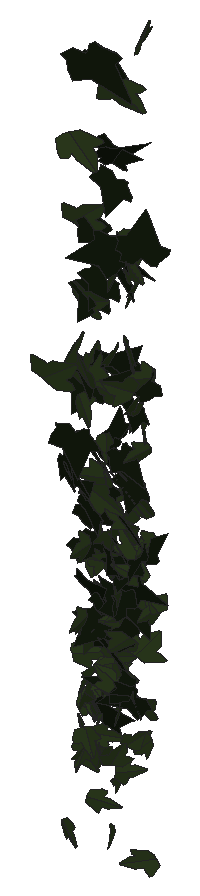
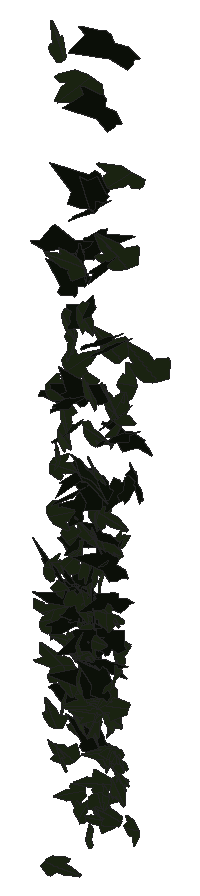
# SketchUp Ruby script. Lengths in inches.
U = 1.inch
M = Sketchup.active_model
def pt(a) = Geom::Point3d.new(a.map { |v| v * U })
def face(e, loops, mat)
  f = e.add_face(loops[0].map { |a| pt(a) })
  loops[1..].each { |l| e.add_face(l.map { |a| pt(a) }).erase! }
  f.material = f.back_material = mat if mat
  f
end
# faces: each face lists its corners as indices into pts; further lists are holes
def faces(e, pts, list, mat = nil) = list.each { |f| face(e, (f[0].is_a?(Array) ? f : [f]).map { |l| l.map { |i| pts[i] } }, mat) }
# xy, xz, yz: faces in a plane at the given z, y or x. An outline is a flat list of corners, or four numbers for a rectangle; further outlines are holes
def ring(l) = l.size == 4 ? [[l[0], l[1]], [l[2], l[1]], [l[2], l[3]], [l[0], l[3]]] : l.each_slice(2).to_a
def flat(e, list, mat, &to3) = list.each { |f| face(e, (f[0].is_a?(Array) ? f : [f]).map { |l| ring(l).map { |u, v| to3.(u, v) } }, mat) }
def xy(e, z, list, mat = nil) = flat(e, list, mat) { |x, y| [x, y, z] }
def xz(e, y, list, mat = nil) = flat(e, list, mat) { |x, z| [x, y, z] }
def yz(e, x, list, mat = nil) = flat(e, list, mat) { |y, z| [x, y, z] }
def lines(e, pts, list) = list.each { |a, b| e.add_line(pt(pts[a]), pt(pts[b])) }
# prism: a flat outline (further loops are holes) pulled along v
def prism(e, loops, v, mat = nil)
  f = face(e, loops, mat); d = Geom::Vector3d.new(v.map { |x| x * U })
  f.pushpull(f.normal.samedirection?(d) ? d.length : -d.length)
end
def box(e, o, s, mat = nil) = prism(e, [[o, [o[0] + s[0], o[1], o[2]], [o[0] + s[0], o[1] + s[1], o[2]], [o[0], o[1] + s[1], o[2]]]], [0, 0, s[2]], mat)
def at(x, y, z, deg = 0) = Geom::Transformation.translation(pt([x, y, z])) * Geom::Transformation.rotation(ORIGIN, Z_AXIS, deg.degrees)
def axes(o, x, y, z) = Geom::Transformation.new([*x, 0, *y, 0, *z, 0, *pt(o).to_a, 1])
def part(name) = M.definitions.add(name)
# library, detail: a bought-in or finely detailed component or shape, given as its bounding box
def library(name, o, s) = part(name).tap { |d| box(d.entities, o, s) }
def detail(e, o, s) = box(e.add_group.entities, o, s)
def put(e, d, t, mat = nil) = e.add_instance(d, t).tap { |i| i.material = mat if mat }
def group(e, t, mat = nil) = e.add_group.tap { |g| g.transformation = t; g.material = mat if mat }.entities
root = M.entities
M.materials.add("1026 AP 7946 SUNNY SIDE UP").color = [254, 231, 186]
M.materials.add("efeu1").color = [18, 25, 13]
M.materials.add("efeu2").color = [43, 57, 29]
c1 = part("ivyleaf_10")
p = [[0,0.5,-0.03],[-0.0625,2.02,-0.43],[-0.19,2.01,-0.46],[-0.54,1.05,-0.29],[-0.52,0.625,-0.18],[-0.83,0.76,-0.28],
  [-1.16,0.64,-0.33],[-1.15,0.33,-0.24],[-0.77,-0.39,0.02],[-0.3,-0.51,0.16],[0.04,-0.48,0.23],[-0.02,2.01,-0.4375],
  [-0.06,2.01,-0.43],[0.04,-0.49,0.23],[0.67,-0.49,0.14],[1.38,0.36,-0.2],[1.375,0.51,-0.24],[0.81,0.65,-0.19],
  [0.62,0.59,-0.15],[0.6,1.09,-0.28],[0.5,1.23,-0.31]]
faces(c1.entities,p,[[0,1,2,3,4,5,6,7,8,9,10],[11,12,0,13,14,15,16,17,18,19,20]],"efeu2")
c2 = part("ivyleaf_9")
p = [[1.54,2.16,1.25],[1.36,2.04,1.19],[-0.21,0.99,0.68],[-0.71,1.11,0.82],[-0.85,0.86,0.67],[-0.8,0.17,0.21],
  [-0.9,-0.01,0.1],[-0.67,-0.16,-0.02],[-0.08,-0.08,-0.05],[-0.03,-0.6,-0.4],[0.65,-0.88,-0.66],[0.83,-0.6,-0.49],
  [1.29,-0.42,-0.43],[1.8125,-0.07,-0.26],[1.21,0.44,0.15]]
faces(c2.entities,p,[[0,1,2,3,4,5,6,7,8,9,10,11,12,13,14]],"efeu1")
put(root,c1,axes([104.67,210.25,259.6],[-0.39071,-0.04225,0.21205],[0.30866,0.06806,0.25862],[-0.11888,0.31556,-0.02542]),"1026 AP 7946 SUNNY SIDE UP")
put(root,c1,axes([104.85,210.58,248.98],[-0.13045,0.07841,-0.19526],[0.16908,-0.15804,-0.1165],[-0.27541,-0.13416,0.02097]),"1026 AP 7946 SUNNY SIDE UP")
put(root,c2,axes([105.08,210.6,258.22],[-0.31451,-0.09252,-0.20284],[0.30315,0.047,-0.22484],[0.15687,-0.27633,0.02783]),"1026 AP 7946 SUNNY SIDE UP")
put(root,c1,axes([105.19,210.78,255.5625],[-0.0292,0.01458,0.27031],[0.11932,-0.25145,0.01847],[0.39547,0.07694,0.01439]),"1026 AP 7946 SUNNY SIDE UP")
put(root,c2,axes([105.41,210.61,267.22],[-0.07439,-0.12984,-0.33099],[0.41359,0.19657,-0.12086],[0.35311,-0.25759,0.07184]),"1026 AP 7946 SUNNY SIDE UP")
put(root,c1,axes([106.08,210.62,250.9],[-0.19009,-0.18862,0.0504],[0.02785,0.04797,0.23082],[-0.30557,0.12171,-0.01032]),"1026 AP 7946 SUNNY SIDE UP")
put(root,c1,axes([106.22,210.9,259.51],[-0.09492,-0.10563,-0.25333],[-0.24533,-0.19017,0.1228],[-0.34084,0.16629,-0.01784]),"1026 AP 7946 SUNNY SIDE UP")
put(root,c2,axes([104.53,210.9,257.35],[-0.01055,-0.07019,-0.26013],[0.39949,-0.06221,0.01051],[-0.09865,-0.2444,0.07039]),"1026 AP 7946 SUNNY SIDE UP")
put(root,c1,axes([105.5,210.8,256.85],[0.07563,0.0111,0.27061],[0.41267,-0.01686,-0.04888],[0.02296,0.26645,-0.0128]),"1026 AP 7946 SUNNY SIDE UP")
put(root,c2,axes([105.71,211.02,262.58],[-0.01995,-0.17839,-0.27056],[0.05025,-0.26121,0.18036],[-0.49535,-0.01931,0.02919]),"1026 AP 7946 SUNNY SIDE UP")
put(root,c2,axes([104.72,210.85,257.2],[0.2917,-0.16938,-0.08061],[-0.10055,0.0445,-0.25833],[0.27493,0.19598,-0.00895]),"1026 AP 7946 SUNNY SIDE UP")
put(root,c1,axes([105.6,211.15,248.78],[0.01372,-0.00257,0.2245],[0.18259,-0.18452,-0.00811],[0.29002,0.1163,-0.00551]),"1026 AP 7946 SUNNY SIDE UP")
put(root,c1,axes([104.72,211.27,253.47],[0.00942,-0.01726,0.24563],[0.11612,-0.22681,-0.02015],[0.35767,0.07409,0.00007]),"1026 AP 7946 SUNNY SIDE UP")
put(root,c1,axes([104.9,211.15,250.91],[0.28899,-0.02084,0.13185],[0.19382,-0.0415,-0.18938],[0.06389,0.22015,-0.02187]),"1026 AP 7946 SUNNY SIDE UP")
put(root,c1,axes([104.86,211.15,250.57],[0.28019,-0.1356,0.01598],[0.00399,-0.02348,-0.23015],[0.21472,0.17739,-0.01658]),"1026 AP 7946 SUNNY SIDE UP")
put(root,c1,axes([105.77,211.08,266.39],[-0.37776,-0.1049,-0.18914],[0.27999,0.04784,-0.26879],[0.17781,-0.29819,0.02141]),"1026 AP 7946 SUNNY SIDE UP")
put(root,c1,axes([104.83,211.125,258.67],[-0.03331,0.2618,0.0245],[-0.00537,0.0221,-0.27045],[-0.41311,-0.02139,0.00154]),"1026 AP 7946 SUNNY SIDE UP")
put(root,c1,axes([106.01,211.14,260.35],[-0.23991,0.22338,0.0069],[-0.02477,-0.00419,-0.27825],[-0.35047,-0.15261,0.01494]),"1026 AP 7946 SUNNY SIDE UP")
put(root,c2,axes([106.13,211.23,252.16],[0.02174,-0.00557,-0.25392],[-0.30638,-0.15144,-0.00862],[-0.23742,0.19492,-0.01212]),"1026 AP 7946 SUNNY SIDE UP")
put(root,c1,axes([104.59,211.03,259.67],[0.10621,-0.15859,0.25953],[-0.13424,0.23812,0.17877],[-0.44967,-0.10854,0.00793]),"1026 AP 7946 SUNNY SIDE UP")
put(root,c1,axes([104.57,211.18,264.68],[0.33939,0.14432,0.17421],[0.24991,0.06302,-0.2653],[-0.24303,0.26634,-0.02953]),"1026 AP 7946 SUNNY SIDE UP")
put(root,c1,axes([104.77,211.3,250.38],[0.01574,-0.23389,0.04801],[0.00412,-0.04787,-0.24145],[0.37538,0.01033,0.00064]),"1026 AP 7946 SUNNY SIDE UP")
put(root,c1,axes([104.92,211.125,251.86],[0.00604,-0.15577,-0.18379],[0.04217,0.17668,-0.15808],[0.36895,-0.01765,0.02108]),"1026 AP 7946 SUNNY SIDE UP")
put(root,c1,axes([105.82,211.31,253.35],[-0.24966,-0.07644,0.13494],[-0.16673,-0.08049,-0.18069],[0.17132,-0.18974,0.0208]),"1026 AP 7946 SUNNY SIDE UP")
put(root,c1,axes([105.56,211.31,252.22],[0.14756,0.18616,0.1326],[-0.10792,-0.10817,0.21385],[0.33812,-0.11576,0.01039]),"1026 AP 7946 SUNNY SIDE UP")
put(root,c1,axes([105.05,211.24,249.4],[-0.03261,-0.03409,-0.20746],[0.31874,0.01972,-0.02485],[0.03675,-0.20129,0.03147]),"1026 AP 7946 SUNNY SIDE UP")
put(root,c2,axes([105.83,211.27,252.21],[-0.24014,0.0961,0.17319],[-0.24571,0.0641,-0.18422],[-0.17854,-0.21747,0.0206]),"1026 AP 7946 SUNNY SIDE UP")
put(root,c1,axes([106.15,211.21,252.0625],[-0.1781,0.18411,0.12725],[-0.12095,0.09621,-0.22171],[-0.32598,-0.13629,0.01274]),"1026 AP 7946 SUNNY SIDE UP")
put(root,c1,axes([104.76,211.32,259.1],[-0.39005,0.11307,-0.08509],[-0.10168,0.05798,0.28002],[0.19596,0.25515,-0.02406]),"1026 AP 7946 SUNNY SIDE UP")
put(root,c2,axes([105.47,211.51,262.44],[0.04387,-0.07054,-0.26418],[0.3938,-0.07866,0.04998],[-0.13892,-0.24524,0.05826]),"1026 AP 7946 SUNNY SIDE UP")
put(root,c1,axes([105.58,211.51,251.76],[0.15613,-0.15263,0.183],[0.12893,-0.15908,-0.18804],[0.34606,0.12813,-0.01251]),"1026 AP 7946 SUNNY SIDE UP")
put(root,c1,axes([105.76,211.5,262.06],[-0.10086,0.00186,-0.26934],[0.24674,-0.21506,-0.04249],[-0.32885,-0.16193,0.05073]),"1026 AP 7946 SUNNY SIDE UP")
put(root,c1,axes([105.34,211.46,252.43],[0.25706,-0.08457,0.11464],[0.14138,-0.06843,-0.18924],[0.16904,0.18583,-0.01606]),"1026 AP 7946 SUNNY SIDE UP")
put(root,c1,axes([104.74,211.55,252.11],[0.06146,-0.1705,0.16311],[0.04199,-0.15719,-0.18099],[0.36449,0.04686,-0.00665]),"1026 AP 7946 SUNNY SIDE UP")
put(root,c1,axes([104.57,211.36,262.75],[-0.32078,-0.12877,0.17326],[0.19886,0.11452,0.24796],[-0.26831,0.23882,-0.02336]),"1026 AP 7946 SUNNY SIDE UP")
put(root,c2,axes([105.34,211.54,252.75],[0.21758,-0.21418,0.00234],[0.01628,0.01083,0.26232],[-0.33643,-0.13799,0.0142]),"1026 AP 7946 SUNNY SIDE UP")
put(root,c1,axes([104.51,211.47,250.96],[-0.11372,0.15878,-0.10474],[0.05418,-0.09691,-0.18014],[-0.29225,-0.07975,0.00736]),"1026 AP 7946 SUNNY SIDE UP")
put(root,c1,axes([105.09,211.53,257.7],[0.23289,-0.0714,0.14625],[0.17784,-0.08975,-0.1681],[0.17634,0.1848,-0.02363]),"1026 AP 7946 SUNNY SIDE UP")
put(root,c2,axes([105.11,211.51,251.24],[0.0382,-0.00478,0.25809],[0.2486,-0.19502,-0.02077],[0.30573,0.15917,-0.01536]),"1026 AP 7946 SUNNY SIDE UP")
put(root,c2,axes([105.8,211.61,256.9],[-0.09049,-0.23355,0.08295],[-0.01312,-0.08215,-0.24803],[0.38892,-0.05712,0.01093]),"1026 AP 7946 SUNNY SIDE UP")
put(root,c2,axes([105.29,211.63,263.78],[-0.11668,-0.25223,0.08957],[-0.01872,-0.08851,-0.27105],[0.41983,-0.07405,0.01281]),"1026 AP 7946 SUNNY SIDE UP")
put(root,c2,axes([106.21,211.33,262.48],[-0.40718,-0.04558,0.17485],[0.25155,0.06504,0.26943],[-0.11531,0.30286,-0.02965]),"1026 AP 7946 SUNNY SIDE UP")
put(root,c1,axes([104.8125,211.42,259.26],[0.39193,-0.17902,0.03078],[-0.01704,0.03771,0.31539],[-0.28515,-0.24832,0.02346]),"1026 AP 7946 SUNNY SIDE UP")
put(root,c2,axes([104.8125,211.48,262.68],[0.07366,-0.2428,-0.1194],[-0.03524,0.11231,-0.25409],[0.42065,0.05193,-0.00038]),"1026 AP 7946 SUNNY SIDE UP")
put(root,c1,axes([105.68,211.58,255.97],[-0.16017,-0.08066,-0.19101],[-0.25573,-0.08981,0.1321],[-0.18779,0.1911,-0.01698]),"1026 AP 7946 SUNNY SIDE UP")
put(root,c1,axes([105.06,211.58,251.47],[0.1803,-0.17179,0.08103],[0.05117,-0.07383,-0.21279],[0.2933,0.11848,-0.01269]),"1026 AP 7946 SUNNY SIDE UP")
put(root,c2,axes([104.5,211.65,259.19],[0.01047,-0.24314,0.07181],[0.01163,-0.07089,-0.25094],[0.39815,0.00846,0.00544]),"1026 AP 7946 SUNNY SIDE UP")
put(root,c1,axes([105.41,211.64,254.18],[-0.10344,0.08288,0.2105],[0.15793,-0.17801,0.1069],[0.30788,0.11916,0.01588]),"1026 AP 7946 SUNNY SIDE UP")
put(root,c2,axes([105.82,211.46,253.35],[-0.26131,0.15261,0.1024],[-0.13415,0.05233,-0.23142],[-0.25216,-0.18597,0.017]),"1026 AP 7946 SUNNY SIDE UP")
put(root,c2,axes([105.7,211.43,254.03],[-0.34158,-0.01045,-0.13283],[-0.20328,0.02189,0.2228],[0.00349,0.25164,-0.02341]),"1026 AP 7946 SUNNY SIDE UP")
put(root,c2,axes([104.61,211.6875,255.93],[0.03816,-0.20861,0.13079],[0.03687,-0.1262,-0.21696],[0.38319,0.03291,0.00785]),"1026 AP 7946 SUNNY SIDE UP")
put(root,c1,axes([104.49,211.66,253.22],[-0.01141,0.0825,-0.19897],[0.00016,-0.19372,-0.08618],[-0.33092,-0.00294,0.00682]),"1026 AP 7946 SUNNY SIDE UP")
put(root,c2,axes([104.97,211.67,253.32],[-0.34817,-0.11962,0.03396],[-0.02695,-0.03869,-0.25815],[0.19353,-0.2206,0.02515]),"1026 AP 7946 SUNNY SIDE UP")
put(root,c2,axes([104.53,211.71,258.74],[-0.18887,-0.21888,0.08833],[-0.03569,-0.08643,-0.25685],[0.36863,-0.12051,0.02038]),"1026 AP 7946 SUNNY SIDE UP")
put(root,c2,axes([105.47,211.64,256],[0.17146,-0.20273,0.09806],[0.06338,-0.08767,-0.23759],[0.34719,0.11612,-0.00506]),"1026 AP 7946 SUNNY SIDE UP")
put(root,c2,axes([105.4,211.64,256.71],[0.21199,-0.17618,0.12948],[0.09275,-0.11377,-0.22834],[0.32836,0.14588,-0.01909]),"1026 AP 7946 SUNNY SIDE UP")
put(root,c2,axes([105.21,211.72,254.8],[0.17525,-0.13069,-0.18207],[0.19656,-0.1243,0.17591],[-0.28315,-0.16717,0.00943]),"1026 AP 7946 SUNNY SIDE UP")
put(root,c1,axes([105.65,211.58,255.7],[-0.24117,0.05716,0.14748],[0.2179,-0.03627,0.16804],[0.10507,0.20642,-0.00997]),"1026 AP 7946 SUNNY SIDE UP")
put(root,c1,axes([105.02,211.57,256.78],[-0.1124,-0.00188,0.24224],[-0.35248,-0.0737,-0.07124],[0.1117,-0.23446,0.01894]),"1026 AP 7946 SUNNY SIDE UP")
put(root,c1,axes([105.98,211.6,267.26],[0.11827,-0.29639,-0.05099],[0.02936,-0.04458,0.31468],[-0.47116,-0.07718,0.00681]),"1026 AP 7946 SUNNY SIDE UP")
put(root,c2,axes([105.5,211.68,262.01],[0.11049,-0.13601,0.23014],[0.22824,-0.17309,-0.15608],[0.34335,0.15883,0.02969]),"1026 AP 7946 SUNNY SIDE UP")
put(root,c1,axes([104.51,211.59,260.71],[-0.25667,0.01621,0.23957],[0.36576,-0.00551,0.16863],[0.02174,0.28399,-0.00873]),"1026 AP 7946 SUNNY SIDE UP")
put(root,c1,axes([106.16,211.63,248.18],[0.15677,0.0237,-0.20343],[-0.29206,-0.06831,-0.10538],[-0.11241,0.21053,-0.00991]),"1026 AP 7946 SUNNY SIDE UP")
put(root,c1,axes([106.06,211.74,259.39],[0.00268,0.0483,0.256],[-0.01027,-0.24813,0.04834],[0.39749,-0.00674,-0.00047]),"1026 AP 7946 SUNNY SIDE UP")
put(root,c2,axes([104.85,211.69,257.21],[0.1503,-0.15026,0.19586],[0.16935,-0.15777,-0.18433],[0.34251,0.14394,0.00519]),"1026 AP 7946 SUNNY SIDE UP")
put(root,c1,axes([105.91,211.55,258.91],[0.03799,-0.26106,-0.07214],[-0.01595,0.06789,-0.26967],[0.42411,0.02594,-0.00368]),"1026 AP 7946 SUNNY SIDE UP")
put(root,c2,axes([106.09,211.72,259.35],[-0.06432,-0.12249,-0.22488],[-0.15798,-0.19379,0.1307],[-0.35945,0.10709,-0.0172]),"1026 AP 7946 SUNNY SIDE UP")
put(root,c1,axes([105.87,211.66,254.68],[0.10562,0.09858,0.19017],[-0.19959,-0.13421,0.121],[0.26064,-0.14272,0.0156]),"1026 AP 7946 SUNNY SIDE UP")
put(root,c2,axes([104.47,211.67,257.42],[0.25226,-0.2001,0.04438],[0.0214,-0.04562,-0.26386],[0.32152,0.16003,-0.01725]),"1026 AP 7946 SUNNY SIDE UP")
put(root,c1,axes([105.25,211.63,259.76],[0.0692,-0.26731,0.00468],[-0.00569,-0.00673,-0.27909],[0.42039,0.04391,-0.00455]),"1026 AP 7946 SUNNY SIDE UP")
put(root,c2,axes([105.51,211.58,257.51],[0.08607,-0.20152,-0.15844],[-0.04183,0.15073,-0.21394],[0.39532,0.05982,0.01186]),"1026 AP 7946 SUNNY SIDE UP")
put(root,c2,axes([104.63,211.82,260.86],[-0.17164,-0.21798,0.12258],[-0.04753,-0.1187,-0.25068],[0.38853,-0.11082,0.02349]),"1026 AP 7946 SUNNY SIDE UP")
put(root,c1,axes([105.94,211.77,257.65],[-0.02414,-0.09557,0.19933],[-0.04813,-0.1916,-0.10084],[0.33668,-0.03424,-0.00012]),"1026 AP 7946 SUNNY SIDE UP")
put(root,c1,axes([105.53,211.68,262.46],[-0.08159,-0.01667,-0.27051],[0.38147,-0.10639,-0.04307],[-0.15976,-0.24551,0.03532]),"1026 AP 7946 SUNNY SIDE UP")
put(root,c2,axes([105.28,211.57,259.36],[-0.18533,-0.01149,0.24255],[0.36954,-0.02706,0.11965],[0.03004,0.26197,0.02455]),"1026 AP 7946 SUNNY SIDE UP")
put(root,c1,axes([106.13,211.6,256.35],[-0.20303,0.05043,-0.17723],[-0.24993,0.0666,0.14317],[0.13129,0.20477,-0.00152]),"1026 AP 7946 SUNNY SIDE UP")
put(root,c2,axes([105.54,211.73,254.95],[-0.32893,-0.07376,-0.10427],[0.16135,0.0106,-0.22733],[0.11197,-0.23197,0.02127]),"1026 AP 7946 SUNNY SIDE UP")
put(root,c2,axes([104.52,211.76,253.89],[-0.07811,-0.04816,0.24698],[0.20339,-0.21309,-0.01772],[0.3268,0.12111,0.07005]),"1026 AP 7946 SUNNY SIDE UP")
put(root,c1,axes([105.77,211.58,250.79],[-0.13261,-0.13051,0.13696],[0.09307,0.12046,0.16032],[-0.27865,0.10235,-0.01163]),"1026 AP 7946 SUNNY SIDE UP")
put(root,c2,axes([105.24,211.82,255.13],[0.00292,-0.1314,0.22313],[0.0885,-0.21173,-0.1336],[0.38941,0.0491,0.02869]),"1026 AP 7946 SUNNY SIDE UP")
put(root,c1,axes([106.12,211.64,250.93],[0.21967,-0.15689,-0.09427],[-0.11693,0.05469,-0.21534],[0.25978,0.15728,-0.01721]),"1026 AP 7946 SUNNY SIDE UP")
put(root,c1,axes([105.35,211.78,253.4375],[-0.01498,0.04787,0.2089],[-0.07479,-0.19786,0.04472],[0.31854,-0.0442,0.02032]),"1026 AP 7946 SUNNY SIDE UP")
put(root,c2,axes([105.68,211.68,254.07],[-0.02695,-0.21843,-0.13728],[0.04767,0.12964,-0.22426],[0.39848,-0.03028,0.01754]),"1026 AP 7946 SUNNY SIDE UP")
put(root,c1,axes([106.16,211.84,253.94],[-0.05313,-0.02706,0.23788],[0.04987,-0.23184,-0.02455],[0.36239,0.02794,0.03826]),"1026 AP 7946 SUNNY SIDE UP")
put(root,c1,axes([105.3,211.82,249.7],[-0.03522,-0.06502,-0.2015],[-0.04332,-0.19366,0.06857],[-0.32064,0.03331,0.01287]),"1026 AP 7946 SUNNY SIDE UP")
put(root,c2,axes([105.59,211.67,254.42],[0.16562,-0.01763,-0.22767],[0.31958,0.10515,0.09181],[0.13886,-0.22098,0.06026]),"1026 AP 7946 SUNNY SIDE UP")
put(root,c1,axes([105.46,211.8125,253.62],[-0.0232,-0.04882,0.20844],[-0.07414,-0.19707,-0.05361],[0.31921,-0.04932,0.0027]),"1026 AP 7946 SUNNY SIDE UP")
put(root,c2,axes([104.82,211.7,256.42],[-0.15752,-0.07194,-0.22236],[0.30103,0.09995,-0.12551],[0.19217,-0.21554,0.01435]),"1026 AP 7946 SUNNY SIDE UP")
put(root,c2,axes([105.63,211.86,258.53],[-0.04582,-0.19985,0.14158],[0.02195,-0.1407,-0.20685],[0.38175,-0.0159,0.02889]),"1026 AP 7946 SUNNY SIDE UP")
put(root,c1,axes([104.87,211.81,256.74],[-0.00763,-0.009,0.21925],[0.22381,-0.15859,-0.00449],[0.24931,0.14209,0.01074]),"1026 AP 7946 SUNNY SIDE UP")
put(root,c1,axes([104.66,211.64,251.35],[-0.26892,0.14404,0.02674],[-0.04963,0.0014,-0.22949],[-0.22449,-0.17286,0.0187]),"1026 AP 7946 SUNNY SIDE UP")
put(root,c1,axes([105.16,211.66,255.48],[-0.1029,-0.23676,-0.05125],[0.02499,0.04582,-0.25277],[0.37916,-0.06728,0.00275]),"1026 AP 7946 SUNNY SIDE UP")
put(root,c2,axes([105.36,211.65,257.74],[-0.22547,0.2023,-0.00715],[-0.01055,-0.01465,-0.25514],[-0.31818,-0.14287,0.01352]),"1026 AP 7946 SUNNY SIDE UP")
put(root,c1,axes([105.77,211.7,255.25],[0.19137,0.22637,0.07581],[-0.07945,-0.05473,0.26381],[0.36511,-0.13056,0.01767]),"1026 AP 7946 SUNNY SIDE UP")
put(root,c1,axes([106.02,211.72,251.6],[-0.28979,0.04874,0.10891],[0.16925,-0.00272,0.19509],[0.06869,0.21231,-0.0212]),"1026 AP 7946 SUNNY SIDE UP")
put(root,c1,axes([105.04,211.66,252.3],[-0.1436,-0.05156,-0.23233],[0.35461,0.0328,-0.10175],[0.07904,-0.24082,0.03438]),"1026 AP 7946 SUNNY SIDE UP")
put(root,c1,axes([105.51,211.5625,250.06],[-0.00453,-0.02696,-0.22851],[0.22295,0.17103,-0.02233],[0.27123,-0.14104,0.01453]),"1026 AP 7946 SUNNY SIDE UP")
put(root,c2,axes([105.73,211.8,255.29],[-0.27608,0.00545,-0.17906],[0.26883,-0.03998,-0.17941],[-0.05024,-0.24382,0.02395]),"1026 AP 7946 SUNNY SIDE UP")
put(root,c1,axes([104.4,211.59,252.43],[0.07217,-0.00443,-0.23803],[0.30938,0.12427,0.03854],[0.19053,-0.2001,0.02758]),"1026 AP 7946 SUNNY SIDE UP")
put(root,c1,axes([104.38,211.76,251.22],[0.11777,0.0083,0.21208],[0.32055,-0.03437,-0.0752],[0.04641,0.21631,-0.01879]),"1026 AP 7946 SUNNY SIDE UP")
put(root,c1,axes([105.05,211.74,256.24],[0.21336,-0.08832,-0.14337],[0.20079,-0.05662,0.16555],[-0.16281,-0.18556,0.01629]),"1026 AP 7946 SUNNY SIDE UP")
put(root,c1,axes([104.92,211.79,256.33],[0.17234,-0.18381,0.05971],[0.0268,-0.05837,-0.22029],[0.30236,0.10994,-0.01451]),"1026 AP 7946 SUNNY SIDE UP")
put(root,c1,axes([104.85,211.74,250.22],[-0.1615,-0.19463,0.02244],[-0.00208,-0.02515,-0.2266],[0.30813,-0.10218,0.01023]),"1026 AP 7946 SUNNY SIDE UP")
put(root,c2,axes([105.04,211.62,264.28],[0.25363,0.22666,-0.07874],[0.04771,0.07361,0.28647],[0.37374,-0.16321,0.01687]),"1026 AP 7946 SUNNY SIDE UP")
put(root,c2,axes([104.95,211.8,264.26],[0.05154,-0.03931,0.26664],[0.29853,-0.17636,-0.05335],[0.28394,0.19256,0.00769]),"1026 AP 7946 SUNNY SIDE UP")
put(root,c2,axes([104.73,211.74,266.48],[-0.0083,-0.03365,-0.30761],[0.4238,0.13107,-0.01937],[0.20821,-0.26813,0.02717]),"1026 AP 7946 SUNNY SIDE UP")
put(root,c1,axes([105.73,211.86,258.5],[0.09492,-0.19843,0.13334],[0.07099,-0.12267,-0.21429],[0.36669,0.07511,0.00697]),"1026 AP 7946 SUNNY SIDE UP")
put(root,c1,axes([105.18,211.69,258.7],[0.02383,0.0299,0.22217],[-0.34039,0.02352,0.01246],[-0.03396,-0.21474,0.03101]),"1026 AP 7946 SUNNY SIDE UP")
put(root,c1,axes([106.23,211.73,254.1],[0.24803,0.06857,0.15658],[-0.23546,-0.03258,0.17549],[0.11407,-0.21634,0.02178]),"1026 AP 7946 SUNNY SIDE UP")
put(root,c1,axes([104.6875,211.78,256.23],[0.33298,0.01177,-0.01381],[-0.01925,-0.02137,-0.21759],[-0.02052,0.21112,-0.02]),"1026 AP 7946 SUNNY SIDE UP")
put(root,c2,axes([105.17,211.64,254.99],[0.11351,-0.04746,-0.24172],[-0.34842,0.07874,-0.08628],[0.14132,0.23224,-0.01857]),"1026 AP 7946 SUNNY SIDE UP")
put(root,c1,axes([104.8,211.69,254.71],[0.12804,-0.08688,-0.18425],[-0.22392,0.10863,-0.12086],[0.21719,0.16322,-0.01599]),"1026 AP 7946 SUNNY SIDE UP")
put(root,c1,axes([105.93,211.67,252.98],[0.36315,0.01849,-0.13478],[0.19613,0.05699,0.23529],[0.06901,-0.25929,0.04051]),"1026 AP 7946 SUNNY SIDE UP")
put(root,c1,axes([105.14,211.72,252.53],[-0.17921,-0.01587,0.19887],[0.28343,0.07357,0.11624],[-0.11186,0.21184,-0.02408]),"1026 AP 7946 SUNNY SIDE UP")
put(root,c2,axes([104.47,211.72,255.83],[0.11885,-0.0334,-0.24162],[0.29729,0.15654,0.04075],[0.22397,-0.19007,0.07412]),"1026 AP 7946 SUNNY SIDE UP")
put(root,c1,axes([105.22,211.92,252.89],[0.03329,-0.01254,0.23383],[0.18352,-0.1951,-0.02346],[0.30687,0.11804,-0.01134]),"1026 AP 7946 SUNNY SIDE UP")
put(root,c1,axes([104.58,211.75,251.41],[0.24473,0.16639,0.02366],[0.0413,0.00551,-0.23415],[-0.26066,0.1571,-0.01489]),"1026 AP 7946 SUNNY SIDE UP")
put(root,c1,axes([105.25,211.79,254.83],[-0.34543,-0.12747,0.05691],[-0.05759,-0.04796,-0.2609],[0.2112,-0.22157,0.02194]),"1026 AP 7946 SUNNY SIDE UP")
put(root,c2,axes([105.73,211.94,259.2],[-0.03043,-0.21024,-0.12331],[-0.0262,-0.11743,0.21675],[-0.37857,0.02503,-0.00509]),"1026 AP 7946 SUNNY SIDE UP")
put(root,c1,axes([104.5625,211.88,250.44],[-0.08991,0.09504,-0.1813],[0.11271,-0.16173,-0.11458],[-0.2944,-0.09095,0.0115]),"1026 AP 7946 SUNNY SIDE UP")
put(root,c1,axes([104.6,211.66,252.8],[-0.02232,-0.12851,-0.19569],[0.09621,0.18055,-0.12999],[0.34656,-0.0584,0.02348]),"1026 AP 7946 SUNNY SIDE UP")
put(root,c1,axes([104.42,211.78,249.91],[0.10583,-0.02682,-0.19811],[0.30389,-0.00854,0.07092],[-0.0267,-0.20342,0.02193]),"1026 AP 7946 SUNNY SIDE UP")
put(root,c2,axes([104.43,211.71,255.03],[0.07648,-0.10723,-0.22267],[0.08856,0.21886,-0.0978],[0.36803,-0.03038,0.0698]),"1026 AP 7946 SUNNY SIDE UP")
put(root,c2,axes([105.09,211.97,261.51],[0.09894,-0.21728,0.16054],[0.08885,-0.14697,-0.23362],[0.4121,0.08385,0.01182]),"1026 AP 7946 SUNNY SIDE UP")
put(root,c1,axes([105,211.64,251.93],[0.01466,-0.06977,-0.24227],[0.00969,0.23494,-0.0703],[0.38499,-0.00325,0.01099]),"1026 AP 7946 SUNNY SIDE UP")
put(root,c1,axes([105.22,211.7,253.84],[-0.0857,0.04001,-0.2584],[-0.30318,0.16084,0.07047],[0.26054,0.20033,-0.00299]),"1026 AP 7946 SUNNY SIDE UP")
put(root,c1,axes([105.2,211.96,253.78],[-0.00636,-0.03454,0.20744],[0.1475,-0.17944,-0.03079],[0.28572,0.09187,0.02051]),"1026 AP 7946 SUNNY SIDE UP")
put(root,c1,axes([104.54,211.72,251.38],[0.00785,-0.07255,-0.22255],[0.30322,0.11576,-0.03485],[0.18977,-0.18197,0.0649]),"1026 AP 7946 SUNNY SIDE UP")
put(root,c2,axes([104.72,212.02,261.08],[-0.18367,-0.21538,0.09808],[-0.02942,-0.09881,-0.25127],[0.36989,-0.11481,0.02872]),"1026 AP 7946 SUNNY SIDE UP")
put(root,c1,axes([104.76,211.72,250.59],[0.00512,0.01748,0.21972],[0.21085,0.16594,-0.01516],[-0.26203,0.13387,-0.0079]),"1026 AP 7946 SUNNY SIDE UP")
put(root,c1,axes([105.65,211.87,252.95],[-0.3121,-0.12444,0.06502],[-0.06646,-0.05225,-0.24067],[0.20962,-0.20184,0.0205]),"1026 AP 7946 SUNNY SIDE UP")
put(root,c1,axes([104.54,211.86,254.65],[0.30341,0.0873,0.00368],[0.01636,-0.01556,-0.21745],[-0.13638,0.19236,-0.0179]),"1026 AP 7946 SUNNY SIDE UP")
put(root,c1,axes([105.92,212.02,255.36],[-0.03371,-0.05562,0.24108],[0.07621,-0.23144,-0.05338],[0.37095,0.04249,0.03288]),"1026 AP 7946 SUNNY SIDE UP")
put(root,c1,axes([105.58,211.91,261.28],[0.10391,-0.21644,0.05244],[0.0158,-0.05142,-0.23337],[0.3497,0.06663,-0.00504]),"1026 AP 7946 SUNNY SIDE UP")
put(root,c2,axes([104.96,211.7,252.94],[0.12299,0.11158,-0.21323],[0.12985,0.19191,0.13942],[0.34712,-0.11132,0.0234]),"1026 AP 7946 SUNNY SIDE UP")
put(root,c1,axes([104.85,211.7,255.27],[-0.03207,0.10184,-0.19221],[-0.07178,0.18156,0.10796],[0.32726,0.0498,0.00484]),"1026 AP 7946 SUNNY SIDE UP")
put(root,c1,axes([105.25,211.83,253.74],[-0.02135,-0.03795,-0.23367],[0.3611,-0.00921,-0.01264],[-0.01109,-0.22682,0.03824]),"1026 AP 7946 SUNNY SIDE UP")
put(root,c1,axes([105.12,211.96,261.58],[0.05462,-0.24999,0.11305],[0.03924,-0.10869,-0.26048],[0.4284,0.04183,0.00944]),"1026 AP 7946 SUNNY SIDE UP")
put(root,c1,axes([105.74,211.98,258.04],[-0.05211,0.07448,-0.2053],[0.10032,-0.18938,-0.08477],[-0.31979,-0.07155,0.00686]),"1026 AP 7946 SUNNY SIDE UP")
put(root,c2,axes([105.25,211.68,257.78],[-0.26579,0.13084,-0.12712],[-0.13207,0.09345,0.21984],[0.25097,0.18774,-0.01893]),"1026 AP 7946 SUNNY SIDE UP")
put(root,c2,axes([105.93,211.85,255.18],[-0.10289,0.15921,0.17797],[0.1246,-0.15287,0.17609],[0.34664,0.10221,-0.01047]),"1026 AP 7946 SUNNY SIDE UP")
put(root,c1,axes([104.96,211.72,252.14],[0.17081,0.00169,-0.21075],[0.23447,0.15793,0.08383],[0.22025,-0.16944,0.07419]),"1026 AP 7946 SUNNY SIDE UP")
put(root,c2,axes([104.65,211.77,252.93],[0.07078,0.2379,0.00813],[-0.01785,-0.0045,0.24918],[0.37379,-0.04526,0.01036]),"1026 AP 7946 SUNNY SIDE UP")
put(root,c2,axes([104.97,211.75,253.9375],[0.03103,-0.04609,-0.25755],[0.05921,0.24825,-0.04268],[0.3949,-0.0336,0.02664]),"1026 AP 7946 SUNNY SIDE UP")
